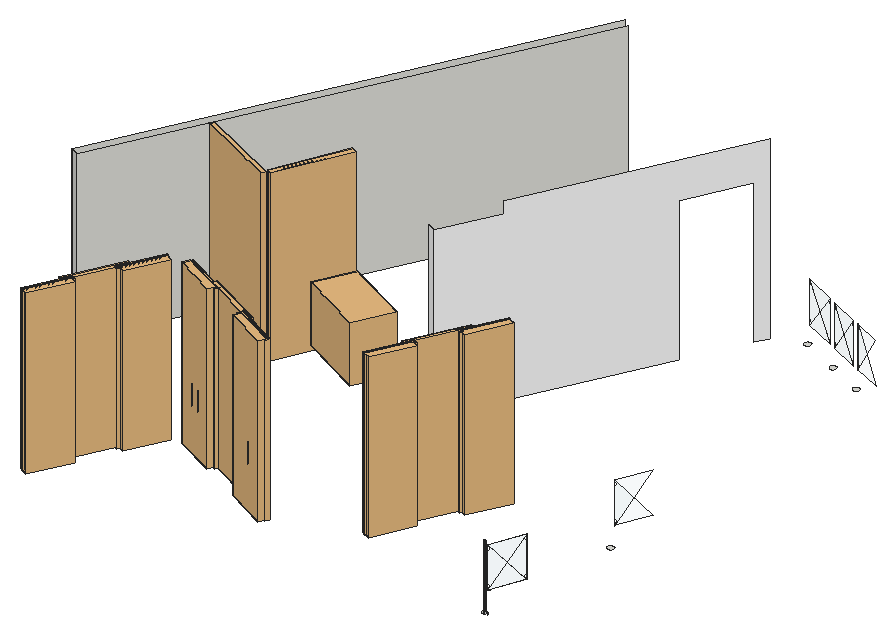
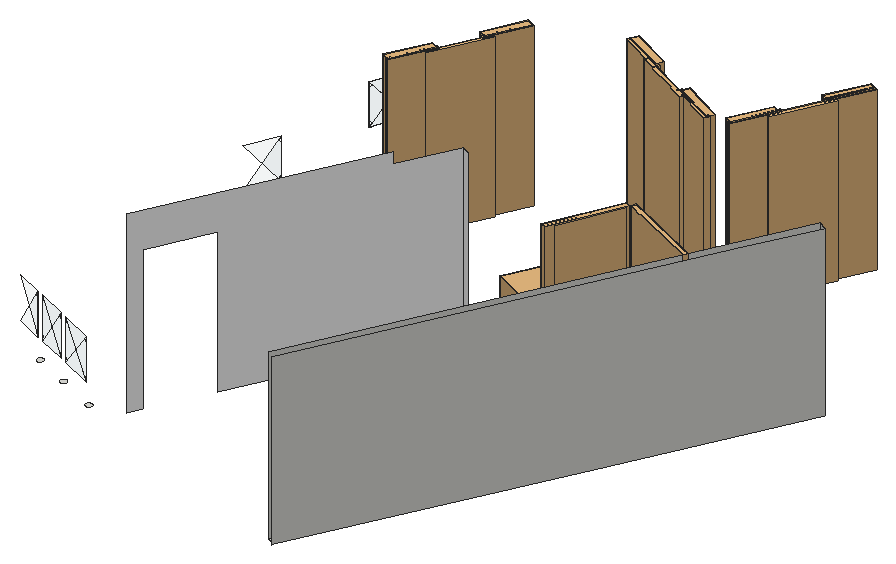
# SketchUp Ruby script. Lengths in inches.
U = 1.inch
M = Sketchup.active_model
def pt(a) = Geom::Point3d.new(a.map { |v| v * U })
def face(e, loops, mat)
  f = e.add_face(loops[0].map { |a| pt(a) })
  loops[1..].each { |l| e.add_face(l.map { |a| pt(a) }).erase! }
  f.material = f.back_material = mat if mat
  f
end
# faces: each face lists its corners as indices into pts; further lists are holes
def faces(e, pts, list, mat = nil) = list.each { |f| face(e, (f[0].is_a?(Array) ? f : [f]).map { |l| l.map { |i| pts[i] } }, mat) }
# xy, xz, yz: faces in a plane at the given z, y or x. An outline is a flat list of corners, or four numbers for a rectangle; further outlines are holes
def ring(l) = l.size == 4 ? [[l[0], l[1]], [l[2], l[1]], [l[2], l[3]], [l[0], l[3]]] : l.each_slice(2).to_a
def flat(e, list, mat, &to3) = list.each { |f| face(e, (f[0].is_a?(Array) ? f : [f]).map { |l| ring(l).map { |u, v| to3.(u, v) } }, mat) }
def xy(e, z, list, mat = nil) = flat(e, list, mat) { |x, y| [x, y, z] }
def xz(e, y, list, mat = nil) = flat(e, list, mat) { |x, z| [x, y, z] }
def yz(e, x, list, mat = nil) = flat(e, list, mat) { |y, z| [x, y, z] }
def lines(e, pts, list) = list.each { |a, b| e.add_line(pt(pts[a]), pt(pts[b])) }
# prism: a flat outline (further loops are holes) pulled along v
def prism(e, loops, v, mat = nil)
  f = face(e, loops, mat); d = Geom::Vector3d.new(v.map { |x| x * U })
  f.pushpull(f.normal.samedirection?(d) ? d.length : -d.length)
end
def box(e, o, s, mat = nil) = prism(e, [[o, [o[0] + s[0], o[1], o[2]], [o[0] + s[0], o[1] + s[1], o[2]], [o[0], o[1] + s[1], o[2]]]], [0, 0, s[2]], mat)
def at(x, y, z, deg = 0) = Geom::Transformation.translation(pt([x, y, z])) * Geom::Transformation.rotation(ORIGIN, Z_AXIS, deg.degrees)
def axes(o, x, y, z) = Geom::Transformation.new([*x, 0, *y, 0, *z, 0, *pt(o).to_a, 1])
def part(name) = M.definitions.add(name)
# library, detail: a bought-in or finely detailed component or shape, given as its bounding box
def library(name, o, s) = part(name).tap { |d| box(d.entities, o, s) }
def detail(e, o, s) = box(e.add_group.entities, o, s)
def put(e, d, t, mat = nil) = e.add_instance(d, t).tap { |i| i.material = mat if mat }
def group(e, t, mat = nil) = e.add_group.tap { |g| g.transformation = t; g.material = mat if mat }.entities
root = M.entities
M.materials.add("Aluminum_Blurry").color = [83, 85, 85]
M.materials.add("Glass1").color = [249, 249, 249]
M.materials["Glass1"].alpha = 0.16
M.materials.add("Glass_Safety_01").color = [204, 235, 244]
M.materials["Glass_Safety_01"].alpha = 0.1
M.materials.add("[Color_000]").color = [255, 255, 255]
c1 = library("Group14",[-64.97,9.24,0.31],[138.52,9.93,292.57])
c2 = library("Group16",[86.37,-10.76,76.46],[21.79,14.87,35.97])
c3 = library("Group22",[48.82,-10.91,0.23],[97.72,18.57,293.12])
c4 = library("Group24",[44.03,2.01,0.26],[103.73,11,292.35])
c5 = library("Group27",[-106.21,-10.76,76.46],[21.8,14.87,35.97])
c6 = library("Group35",[-145.81,2.01,0.26],[103.73,11,292.35])
c7 = library("Group33",[-144.59,-10.91,0.23],[97.72,18.57,293.12])
c8 = part("Group\#71")
put(c8.entities,c1,at(145.81,10.91,-0.23))
put(c8.entities,c2,at(145.81,10.91,-0.23))
put(c8.entities,c3,at(145.81,10.91,-0.23))
put(c8.entities,c4,at(145.81,10.91,-0.23))
put(c8.entities,c5,at(145.81,10.91,-0.23))
put(c8.entities,c6,at(145.81,10.91,-0.23))
put(c8.entities,c7,at(145.81,10.91,-0.23))
c9 = library("KOŁO+DRZWI+WNĘKOWE+SKRZYDŁOWE+NEXT+80,+PRAWOSTRONNE+HDRF80R\#",[0.43,0.44,0],[31.07,2.7,98.875])
c10 = library("bathroom kit",[-10.19,-11.89,-0.14],[22.08,39.51,30.77])
c11 = library("Grupa\#6",[0,0,0],[3037.62,97.06,7677.17])
c12 = library("Grupa\#5",[-370.2,0,0],[3507.76,312.85,9902.72])
c13 = part("Grupa\#4")
put(c13.entities,c11,axes([63,67.3,0],[1,0,0],[0,1,0],[0,0,1.28401]),"Glass1")
put(c13.entities,c12,at(0,0,0),"Aluminum_Blurry")
c14 = library("Kohler_Balast_1935.skp\#1",[-38.83,-18.45,0],[74.81,42.21,2.86])
xy(root,321.27,[[671.22,867.45,666.72,869.64,714.3125,967.65,718.8125,965.47],[718.8125,965.47,714.3125,967.65,780.33,1103.61,784.83,1101.43]])
xy(root,321.27,[[729.86,958.59,730.27,958.67,730.63,958.85,730.94,959.125,731.17,959.47,730.32,959.88,730.23,959.74,730.1,959.63,729.96,959.5625,729.8,959.53,729.63,959.54,729.48,959.59,729.34,959.68,729.23,959.8,729.16,959.95,729.12,960.11,729.13,960.28,729.18,960.43,728.33,960.84,728.2,960.45,728.18,960.04,728.26,959.64,728.45,959.27,728.72,958.97,729.0625,958.74,729.45,958.61],[729.8,959.53,729.96,959.5625,730.1,959.63,730.23,959.74,730.32,959.88,729.18,960.43,729.13,960.28,729.12,960.11,729.16,959.95,729.23,959.8,729.34,959.68,729.48,959.59,729.63,959.54]],"[Color_000]")
xy(root,321.86,[[961.92,866.71,962.32,866.79,962.6875,866.97,962.99,867.25,963.22,867.59,963.35,867.98,963.375,868.39,963.29,868.79,963.11,869.16,962.83,869.47,962.49,869.69,962.1,869.82,961.69,869.85,961.29,869.77,960.92,869.58,960.61,869.31,960.39,868.97,960.26,868.58,960.23,868.17,960.32,867.76,960.5,867.4,960.77,867.09,961.12,866.86,961.51,866.73],[957.4375,1039.9,957.84,1039.98,958.21,1040.17,958.51,1040.44,958.74,1040.79,958.87,1041.18,958.9,1041.59,958.8125,1041.99,958.63,1042.36,958.36,1042.66,958.01,1042.89,957.62,1043.02,957.21,1043.04,956.81,1042.96,956.44,1042.78,956.13,1042.5,955.91,1042.16,955.78,1041.77,955.75,1041.36,955.84,1040.96,956.02,1040.59,956.29,1040.28,956.64,1040.06,957.03,1039.93],[938.05,1048.34,938.46,1048.43,938.82,1048.61,939.13,1048.88,939.36,1049.23,939.49,1049.62,939.51,1050.03,939.43,1050.43,939.25,1050.8,938.97,1051.11,938.63,1051.33,938.24,1051.46,937.83,1051.49,937.43,1051.4,937.06,1051.22,936.75,1050.95,936.52,1050.6,936.4,1050.21,936.37,1049.8,936.45,1049.4,936.64,1049.03,936.91,1048.72,937.25,1048.5,937.64,1048.37],[916.82,1057.59,917.22,1057.67,917.59,1057.86,917.9,1058.13,918.125,1058.47,918.25,1058.86,918.28,1059.28,918.2,1059.68,918.01,1060.05,917.74,1060.35,917.4,1060.58,917.01,1060.71,916.6,1060.73,916.19,1060.65,915.83,1060.47,915.52,1060.19,915.29,1059.85,915.16,1059.46,915.14,1059.05,915.22,1058.65,915.4,1058.28,915.68,1057.97,916.02,1057.75,916.41,1057.62]])
xy(root,331.9,[[955.76,792.12,955.58,792.19,962.85,810.18],[955.58,792.19,962.67,810.25,962.85,810.18],[955.48,1042.17,939.54,1049.11,939.62,1049.29],[955.48,1042.17,939.62,1049.29,955.56,1042.35],[936.1,1050.61,918.32,1058.35,918.4,1058.53],
  [936.1,1050.61,918.4,1058.53,936.18,1050.79]],"Glass_Safety_01")
p = [[953.53,791.01,321.27],[953.4,790.62,321.27],[953.4,790.62,321.86],[953.53,791.01,321.86],[954.6,790.84,321.27],[954.47,790.74,321.27],
  [954.47,790.74,357.27],[954.6,790.84,357.27],[955.47,790.68,321.27],[955.36,790.8,321.27],[955.36,790.8,357.27],[955.47,790.68,357.27],
  [954.74,790.92,321.27],[954.74,790.92,357.27],[955.22,790.89,321.27],[955.22,790.89,357.27],[956.4375,790.84,321.27],[956.25,791.21,321.27],
  [956.25,791.21,321.86],[956.4375,790.84,321.86],[954.9,790.95,321.27],[954.9,790.95,357.27],[955.07,790.94,321.27],[955.07,790.94,357.27],
  [953.76,791.35,321.27],[953.76,791.35,321.86],[955.98,791.51,321.27],[955.98,791.51,321.86],[954.07,791.63,321.27],[954.07,791.63,321.86],
  [955.64,791.74,321.27],[955.64,791.74,321.86],[954.43,791.8125,321.27],[954.43,791.8125,321.86],[955.25,791.87,321.27],[955.25,791.87,321.86],
  [954.84,791.89,321.27],[954.84,791.89,321.86],[666.72,869.64,321.27],[671.22,867.45,321.27],[671.22,867.45,412.84],[666.72,869.64,412.84],
  [718.8125,965.47,321.27],[784.83,1101.43,321.27],[784.83,1101.43,412.84],[686.94,899.84,412.84],[682.44,902.02,412.84],[780.62,1104.21,412.84],
  [780.62,1104.21,321.27],[780.37,1103.68,321.27],[780.33,1103.61,321.27],[714.3125,967.65,321.27],[826.625,913.12,321.27],[831.12,910.93,321.27],
  [831.12,910.93,412.84],[826.625,913.12,412.84],[897.14,1046.9,321.27],[900.47,1053.75,321.27],[900.47,1053.75,418.84],[845.58,940.71,418.84],
  [845.58,940.71,412.84],[881.58,1014.85,321.27],[881.58,1014.85,399.22],[897.14,1046.9,399.22],[955.58,792.19,331.9],[955.76,792.12,331.9],
  [955.76,792.12,333],[955.76,792.12,335.125],[955.76,792.12,351.28],[955.76,792.12,353.41],[955.76,792.12,354.51],[955.58,792.19,354.51],
  [955.58,792.19,353.41],[955.58,792.19,351.28],[955.58,792.19,335.125],[955.58,792.19,333],[955.86,792.375,335.09],[955.95,792.61,334.98],
  [956.03,792.82,334.8125],[956.1,792.98,334.59],[956.14,793.08,334.34],[956.15,793.11,334.0625],[956.14,793.08,333.79],[956.1,792.98,333.53],
  [956.03,792.82,333.3125],[955.95,792.61,333.14],[955.86,792.375,333.04],[962.85,810.18,354.51],[955.86,792.375,353.37],[955.95,792.61,353.27],
  [956.03,792.82,353.1],[956.1,792.98,352.88],[956.14,793.08,352.62],[956.15,793.11,352.35],[956.14,793.08,352.07],[956.1,792.98,351.8125],
  [956.03,792.82,351.59],[955.95,792.61,351.43],[955.86,792.375,351.32],[962.85,810.18,331.9],[962.85,810.18,333],[962.85,810.18,335.125],
  [962.85,810.18,351.28],[962.85,810.18,353.41],[955.68,792.45,333.04],[955.77,792.6875,333.14],[955.85,792.89,333.3125],[955.91,793.05,333.53],
  [955.95,793.15,333.79],[955.97,793.18,334.0625],[955.95,793.15,334.34],[955.91,793.05,334.59],[955.85,792.89,334.8125],[955.77,792.6875,334.98],
  [955.68,792.45,335.09],[955.68,792.45,351.32],[955.77,792.6875,351.43],[955.85,792.89,351.59],[955.91,793.05,351.8125],[955.95,793.15,352.07],
  [955.97,793.18,352.35],[955.95,793.15,352.62],[955.91,793.05,352.88],[955.85,792.89,353.1],[955.77,792.6875,353.27],[955.68,792.45,353.37],
  [962.67,810.25,331.9],[962.67,810.25,351.28],[962.67,810.25,335.125],[962.61,810.09,335.125],[962.51,809.84,335.09],[962.42,809.6,334.98],
  [962.34,809.39,334.8125],[962.27,809.24,334.59],[962.23,809.14,334.34],[962.22,809.1,334.0625],[962.23,809.14,333.79],[962.27,809.24,333.53],
  [962.34,809.39,333.3125],[962.42,809.6,333.14],[962.51,809.84,333.04],[962.61,810.09,333],[962.67,810.25,333],[962.67,810.25,354.51],
  [962.67,810.25,353.41],[962.61,810.09,353.41],[962.51,809.84,353.37],[962.42,809.6,353.27],[962.34,809.39,353.1],[962.27,809.24,352.88],
  [962.23,809.14,352.62],[962.22,809.1,352.35],[962.23,809.14,352.07],[962.27,809.24,351.8125],[962.34,809.39,351.59],[962.42,809.6,351.43],
  [962.51,809.84,351.32],[962.61,810.09,351.28],[962.5,870.12,331.9],[962.68,870.04,331.9],[962.68,870.04,333],[962.68,870.04,335.125],
  [962.68,870.04,351.28],[962.68,870.04,353.41],[962.68,870.04,354.51],[962.5,870.12,354.51],[962.5,870.12,353.41],[962.5,870.12,351.28],
  [962.5,870.12,335.125],[962.5,870.12,333],[962.79,870.3,335.09],[962.89,870.53,334.98],[962.98,870.73,334.8125],[963.05,870.89,334.59],
  [963.09,870.99,334.34],[963.1,871.02,334.0625],[963.09,870.99,333.79],[963.05,870.89,333.53],[962.98,870.73,333.3125],[962.89,870.53,333.14],
  [962.79,870.3,333.04],[970.13,887.16,354.51],[962.79,870.3,353.37],[962.89,870.53,353.27],[962.98,870.73,353.1],[963.05,870.89,352.88],
  [963.09,870.99,352.62],[963.1,871.02,352.35],[963.09,870.99,352.07],[963.05,870.89,351.8125],[962.98,870.73,351.59],[962.89,870.53,351.43],
  [962.79,870.3,351.32],[962.61,870.375,333.04],[962.71,870.61,333.14],[962.8,870.8125,333.3125],[962.87,870.97,333.53],[962.91,871.0625,333.79],
  [962.92,871.1,334.0625],[962.91,871.0625,334.34],[962.87,870.97,334.59],[962.8,870.8125,334.8125],[962.71,870.61,334.98],[962.61,870.375,335.09],
  [962.61,870.375,351.32],[962.71,870.61,351.43],[962.8,870.8125,351.59],[962.87,870.97,351.8125],[962.91,871.0625,352.07],[962.92,871.1,352.35],
  [962.91,871.0625,352.62],[962.87,870.97,352.88],[962.8,870.8125,353.1],[962.71,870.61,353.27],[962.61,870.375,353.37],[969.95,887.24,331.9],
  [958.91,1040.67,351.28],[958.91,1040.67,335.125],[959.09,1040.6,335.125],[959.34,1040.49,335.09],[959.58,1040.38,334.98],[959.78,1040.3,334.8125],
  [959.93,1040.23,334.59],[960.03,1040.1875,334.34],[960.06,1040.17,334.0625],[960.03,1040.1875,333.79],[959.93,1040.23,333.53],[959.78,1040.3,333.3125],
  [959.58,1040.38,333.14],[959.34,1040.49,333.04],[959.09,1040.6,333],[958.91,1040.67,333],[958.91,1040.67,331.9],[973.9375,1034.13,354.51],
  [958.91,1040.67,354.51],[958.91,1040.67,353.41],[959.09,1040.6,353.41],[959.34,1040.49,353.37],[959.58,1040.38,353.27],[959.78,1040.3,353.1],
  [959.93,1040.23,352.88],[960.03,1040.1875,352.62],[960.06,1040.17,352.35],[960.03,1040.1875,352.07],[959.93,1040.23,351.8125],[959.78,1040.3,351.59],
  [959.58,1040.38,351.43],[959.34,1040.49,351.32],[959.09,1040.6,351.28],[958.99,1040.85,331.9],[958.99,1040.85,333],[959.17,1040.78,333],
  [959.42,1040.67,333.04],[959.66,1040.57,333.14],[959.86,1040.48,333.3125],[960.01,1040.41,333.53],[960.11,1040.37,333.79],[960.14,1040.35,334.0625],
  [960.11,1040.37,334.34],[960.01,1040.41,334.59],[959.86,1040.48,334.8125],[959.66,1040.57,334.98],[959.42,1040.67,335.09],[959.17,1040.78,335.125],
  [958.99,1040.85,335.125],[958.99,1040.85,351.28],[959.17,1040.78,351.28],[959.42,1040.67,351.32],[959.66,1040.57,351.43],[959.86,1040.48,351.59],
  [960.01,1040.41,351.8125],[960.11,1040.37,352.07],[960.14,1040.35,352.35],[960.11,1040.37,352.62],[960.01,1040.41,352.88],[959.86,1040.48,353.1],
  [959.66,1040.57,353.27],[959.42,1040.67,353.37],[959.17,1040.78,353.41],[958.99,1040.85,353.41],[958.99,1040.85,354.51],[974.02,1034.3125,331.9],
  [955.48,1042.17,331.9],[955.48,1042.17,333],[955.23,1042.28,333.04],[954.99,1042.38,333.14],[954.79,1042.47,333.3125],[954.64,1042.54,333.53],
  [954.54,1042.58,333.79],[954.51,1042.59,334.0625],[954.54,1042.58,334.34],[954.64,1042.54,334.59],[954.79,1042.47,334.8125],[954.99,1042.38,334.98],
  [955.23,1042.28,335.09],[955.48,1042.17,335.125],[955.48,1042.17,351.28],[955.23,1042.28,351.32],[954.99,1042.38,351.43],[954.79,1042.47,351.59],
  [954.64,1042.54,351.8125],[954.54,1042.58,352.07],[954.51,1042.59,352.35],[954.54,1042.58,352.62],[954.64,1042.54,352.88],[954.79,1042.47,353.1],
  [954.99,1042.38,353.27],[955.23,1042.28,353.37],[955.48,1042.17,353.41],[955.48,1042.17,354.51],[939.54,1049.11,331.9],[939.54,1049.11,351.28],
  [939.54,1049.11,335.125],[939.71,1049.04,335.125],[939.96,1048.93,335.09],[940.19,1048.83,334.98],[940.4,1048.74,334.8125],[940.55,1048.67,334.59],
  [940.65,1048.63,334.34],[940.68,1048.61,334.0625],[940.65,1048.63,333.79],[940.55,1048.67,333.53],[940.4,1048.74,333.3125],[940.19,1048.83,333.14],
  [939.96,1048.93,333.04],[939.71,1049.04,333],[939.54,1049.11,333],[939.54,1049.11,354.51],[939.54,1049.11,353.41],[939.71,1049.04,353.41],
  [939.96,1048.93,353.37],[940.19,1048.83,353.27],[940.4,1048.74,353.1],[940.55,1048.67,352.88],[940.65,1048.63,352.62],[940.68,1048.61,352.35],
  [940.65,1048.63,352.07],[940.55,1048.67,351.8125],[940.4,1048.74,351.59],[940.19,1048.83,351.43],[939.96,1048.93,351.32],[939.71,1049.04,351.28],
  [955.56,1042.35,331.9],[955.56,1042.35,333],[955.56,1042.35,335.125],[955.56,1042.35,351.28],[955.56,1042.35,353.41],[955.56,1042.35,354.51],
  [955.31,1042.46,335.09],[955.07,1042.5625,334.98],[954.87,1042.65,334.8125],[954.72,1042.72,334.59],[954.62,1042.76,334.34],[954.58,1042.77,334.0625],
  [954.62,1042.76,333.79],[954.72,1042.72,333.53],[954.87,1042.65,333.3125],[955.07,1042.5625,333.14],[955.31,1042.46,333.04],[939.62,1049.29,354.51],
  [955.31,1042.46,353.37],[955.07,1042.5625,353.27],[954.87,1042.65,353.1],[954.72,1042.72,352.88],[954.62,1042.76,352.62],[954.58,1042.77,352.35],
  [954.62,1042.76,352.07],[954.72,1042.72,351.8125],[954.87,1042.65,351.59],[955.07,1042.5625,351.43],[955.31,1042.46,351.32],[939.62,1049.29,331.9],
  [939.62,1049.29,333],[939.79,1049.22,333],[940.04,1049.11,333.04],[940.27,1049.01,333.14],[940.47,1048.92,333.3125],[940.63,1048.85,333.53],
  [940.73,1048.81,333.79],[940.76,1048.79,334.0625],[940.73,1048.81,334.34],[940.63,1048.85,334.59],[940.47,1048.92,334.8125],[940.27,1049.01,334.98],
  [940.04,1049.11,335.09],[939.79,1049.22,335.125],[939.62,1049.29,335.125],[939.62,1049.29,351.28],[939.79,1049.22,351.28],[940.04,1049.11,351.32],
  [940.27,1049.01,351.43],[940.47,1048.92,351.59],[940.63,1048.85,351.8125],[940.73,1048.81,352.07],[940.76,1048.79,352.35],[940.73,1048.81,352.62],
  [940.63,1048.85,352.88],[940.47,1048.92,353.1],[940.27,1049.01,353.27],[940.04,1049.11,353.37],[939.79,1049.22,353.41],[939.62,1049.29,353.41],
  [936.1,1050.61,331.9],[936.1,1050.61,333],[935.85,1050.72,333.04],[935.61,1050.82,333.14],[935.41,1050.91,333.3125],[935.25,1050.98,333.53],
  [935.16,1051.02,333.79],[935.12,1051.04,334.0625],[935.16,1051.02,334.34],[935.25,1050.98,334.59],[935.41,1050.91,334.8125],[935.61,1050.82,334.98],
  [935.85,1050.72,335.09],[936.1,1050.61,335.125],[936.1,1050.61,351.28],[935.85,1050.72,351.32],[935.61,1050.82,351.43],[935.41,1050.91,351.59],
  [935.25,1050.98,351.8125],[935.16,1051.02,352.07],[935.12,1051.04,352.35],[935.16,1051.02,352.62],[935.25,1050.98,352.88],[935.41,1050.91,353.1],
  [935.61,1050.82,353.27],[935.85,1050.72,353.37],[936.1,1050.61,353.41],[936.1,1050.61,354.51],[918.32,1058.35,331.9],[918.32,1058.35,351.28],
  [918.32,1058.35,335.125],[918.47,1058.29,335.125],[918.73,1058.18,335.09],[918.96,1058.07,334.98],[919.16,1057.99,334.8125],[919.32,1057.92,334.59],
  [919.42,1057.875,334.34],[919.45,1057.86,334.0625],[919.42,1057.875,333.79],[919.32,1057.92,333.53],[919.16,1057.99,333.3125],[918.96,1058.07,333.14],
  [918.73,1058.18,333.04],[918.47,1058.29,333],[918.32,1058.35,333],[918.32,1058.35,354.51],[918.32,1058.35,353.41],[918.47,1058.29,353.41],
  [918.73,1058.18,353.37],[918.96,1058.07,353.27],[919.16,1057.99,353.1],[919.32,1057.92,352.88],[919.42,1057.875,352.62],[919.45,1057.86,352.35],
  [919.42,1057.875,352.07],[919.32,1057.92,351.8125],[919.16,1057.99,351.59],[918.96,1058.07,351.43],[918.73,1058.18,351.32],[918.47,1058.29,351.28],
  [936.18,1050.79,331.9],[936.18,1050.79,333],[936.18,1050.79,335.125],[936.18,1050.79,351.28],[936.18,1050.79,353.41],[936.18,1050.79,354.51],
  [935.92,1050.9,335.09],[935.6875,1051,334.98],[935.49,1051.09,334.8125],[935.33,1051.16,334.59],[935.23,1051.2,334.34],[935.2,1051.22,334.0625],
  [935.23,1051.2,333.79],[935.33,1051.16,333.53],[935.49,1051.09,333.3125],[935.6875,1051,333.14],[935.92,1050.9,333.04],[918.4,1058.53,354.51],
  [935.92,1050.9,353.37],[935.6875,1051,353.27],[935.49,1051.09,353.1],[935.33,1051.16,352.88],[935.23,1051.2,352.62],[935.2,1051.22,352.35],
  [935.23,1051.2,352.07],[935.33,1051.16,351.8125],[935.49,1051.09,351.59],[935.6875,1051,351.43],[935.92,1050.9,351.32],[918.4,1058.53,331.9],
  [918.4,1058.53,333],[918.55,1058.47,333],[918.8,1058.36,333.04],[919.04,1058.25,333.14],[919.24,1058.17,333.3125],[919.4,1058.1,333.53],
  [919.49,1058.06,333.79],[919.53,1058.04,334.0625],[919.49,1058.06,334.34],[919.4,1058.1,334.59],[919.24,1058.17,334.8125],[919.04,1058.25,334.98],
  [918.8,1058.36,335.09],[918.55,1058.47,335.125],[918.4,1058.53,335.125],[918.4,1058.53,351.28],[918.55,1058.47,351.28],[918.8,1058.36,351.32],
  [919.04,1058.25,351.43],[919.24,1058.17,351.59],[919.4,1058.1,351.8125],[919.49,1058.06,352.07],[919.53,1058.04,352.35],[919.49,1058.06,352.62],
  [919.4,1058.1,352.88],[919.24,1058.17,353.1],[919.04,1058.25,353.27],[918.8,1058.36,353.37],[918.55,1058.47,353.41],[918.4,1058.53,353.41]]
faces(root,p,[[0,1,2,3],[16,17,18,19],[24,0,3,25],[17,26,27,18],[28,24,25,29],[26,30,31,27],[32,28,29,33],[30,34,35,31],
  [34,36,37,35],[38,39,40,41],[39,42,43,44,45,40],[46,47,48,49,50,51,38,41]])
faces(root,p,[[4,5,6,7],[8,9,10,11],[12,4,7,13],[9,14,15,10],[20,12,13,21],[22,20,21,23],[14,22,23,15],[52,53,54,55],
  [56,57,58,59,60,54,53,61,62,63]],"[Color_000]")
faces(root,p,[[64,65,66,67,68,69,70,71,72,73,74,75],[68,67,76,77,78,79,80,81,82,83,84,85,86,66,65,87,70,69,88,89,90,91,92,93,94,95,96,97,98],[87,65,99,100,101,102,103],[64,75,104,105,106,107,108,109,110,111,112,113,114,74,73,115,116,117,118,119,120,121,122,123,124,125,72,71,126],[127,128,129,130,131,132,133,134,135,136,137,138,139,140,141,142,126,71,143,144,145,146,147,148,149,150,151,152,153,154,155,156,157],[99,126,142,128,127,144,143,87,103,102,101,100],[158,159,160,161,162,163,164,165,166,167,168,169],[162,161,170,171,172,173,174,175,176,177,178,179,180,160,159,181,164,163,182,183,184,185,186,187,188,189,190,191,192],
  [158,169,193,194,195,196,197,198,199,200,201,202,203,168,167,204,205,206,207,208,209,210,211,212,213,214,166,165,215],[216,217,218,219,220,221,222,223,224,225,226,227,228,229,230,231,232,233,234,235,236,237,238,239,240,241,242,243,244,245,246,247,248],[249,250,251,252,253,254,255,256,257,258,259,260,261,262,263,264,265,266,267,268,269,270,271,272,273,274,275,276,277,278,279,280,281],[249,232,231,217,216,235,234,280,279,265,264,250],[282,283,284,285,286,287,288,289,290,291,292,293,294,295,296,297,298,299,300,301,302,303,304,305,306,307,308,309,310],[311,312,313,314,315,316,317,318,319,320,321,322,323,324,325,326,310,309,327,328,329,330,331,332,333,334,335,336,337,338,339,340,341],[282,342,343,344,345,346,347,309,308,296,295,283],[345,344,348,349,350,351,352,353,354,355,356,357,358,343,342,359,347,346,360,361,362,363,364,365,366,367,368,369,370],
  [371,372,373,374,375,376,377,378,379,380,381,382,383,384,385,386,387,388,389,390,391,392,393,394,395,396,397,398,399,400,401,359,342],[371,310,326,312,311,328,327,359,401,387,386,372],[402,403,404,405,406,407,408,409,410,411,412,413,414,415,416,417,418,419,420,421,422,423,424,425,426,427,428,429,430],[431,432,433,434,435,436,437,438,439,440,441,442,443,444,445,446,430,429,447,448,449,450,451,452,453,454,455,456,457,458,459,460,461],[402,462,463,464,465,466,467,429,428,416,415,403],[465,464,468,469,470,471,472,473,474,475,476,477,478,463,462,479,467,466,480,481,482,483,484,485,486,487,488,489,490],[491,492,493,494,495,496,497,498,499,500,501,502,503,504,505,506,507,508,509,510,511,512,513,514,515,516,517,518,519,520,521,479,462],[491,430,446,432,431,448,447,479,521,507,506,492]],"Glass_Safety_01")
put(root,c8,axes([729.76,759.02,324.52],[0.10271,0.21152,0],[-0.19887,0.09657,0],[0,0,0.30131]))
put(root,c8,axes([764.56,821.72,324.57],[0.23478,-0.11401,0],[0.09657,0.19887,0],[0,0,0.30131]))
put(root,c8,axes([878.29,806.92,324.52],[0.10271,0.21152,0],[-0.19887,0.09657,0],[0,0,0.30131]))
put(root,c9,axes([743.03,902.71,321.27],[-1.42587,0.63966,0],[0.40931,0.9124,0],[0,0,0.9261]))
put(root,c10,at(777.06,919.64,330.63,-115.9))
put(root,c9,axes([743.62,908.23,321.27],[0.4379,1.00895,0],[0.91733,-0.39813,0],[0,0,0.9261]))
put(root,c13,axes([748.21,909.5625,321.27],[0.0047,0.01057,0],[-0.00917,0.00408,0],[0,0,0.00929]))
put(root,c14,axes([729.3,935.3,321.26],[-0.58251,0.2651,0],[-0.39411,-0.86599,0],[0,0,1]))
